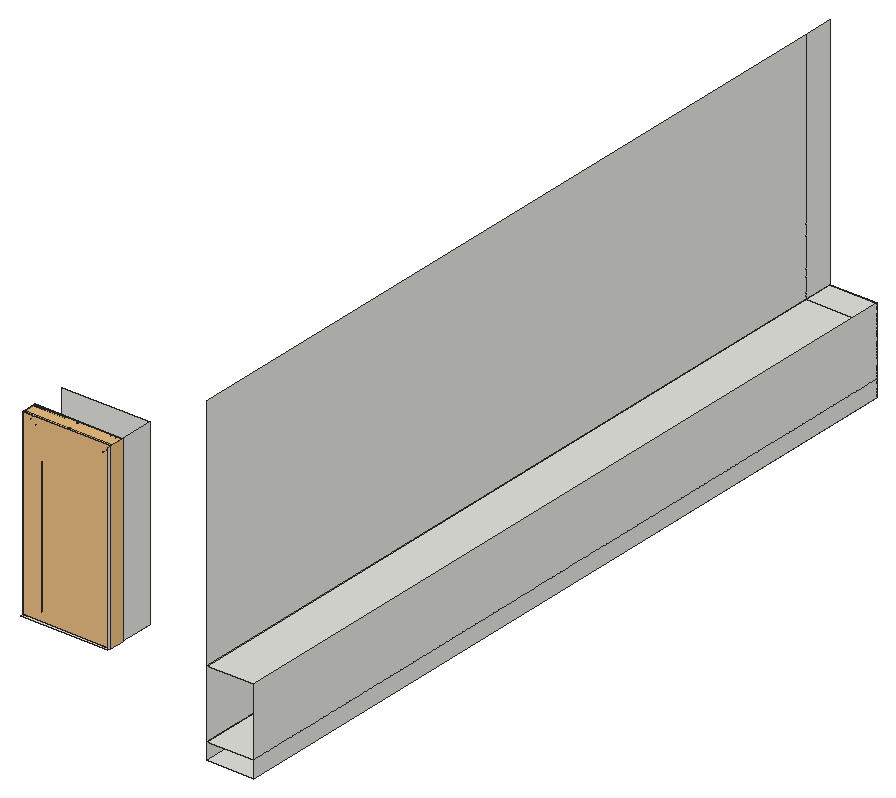
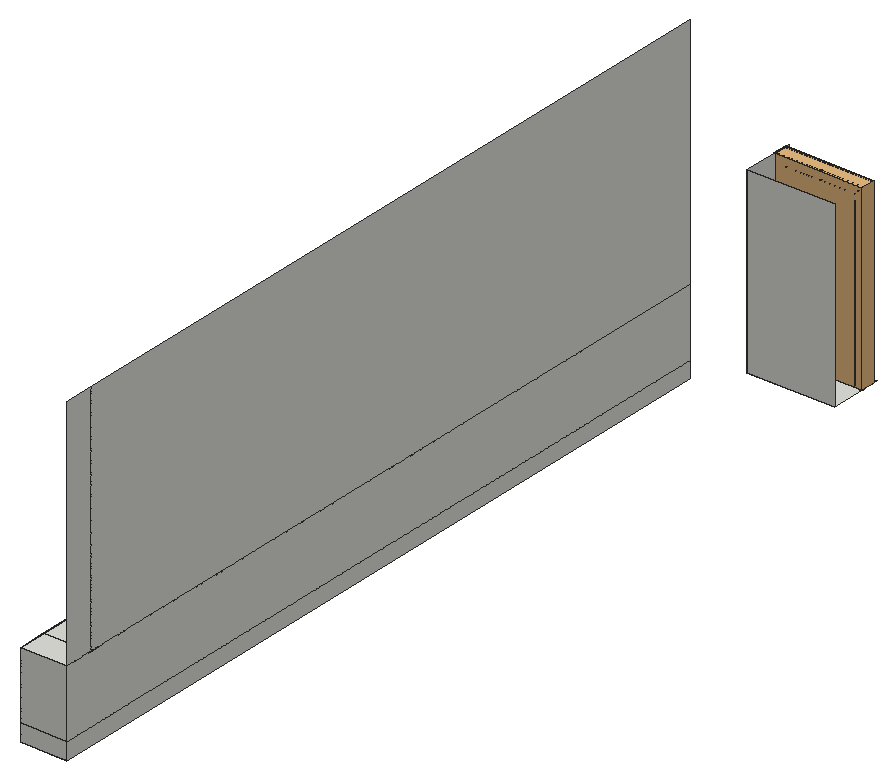
# SketchUp Ruby script. Lengths in inches.
U = 1.inch
M = Sketchup.active_model
def pt(a) = Geom::Point3d.new(a.map { |v| v * U })
def face(e, loops, mat)
  f = e.add_face(loops[0].map { |a| pt(a) })
  loops[1..].each { |l| e.add_face(l.map { |a| pt(a) }).erase! }
  f.material = f.back_material = mat if mat
  f
end
# faces: each face lists its corners as indices into pts; further lists are holes
def faces(e, pts, list, mat = nil) = list.each { |f| face(e, (f[0].is_a?(Array) ? f : [f]).map { |l| l.map { |i| pts[i] } }, mat) }
# xy, xz, yz: faces in a plane at the given z, y or x. An outline is a flat list of corners, or four numbers for a rectangle; further outlines are holes
def ring(l) = l.size == 4 ? [[l[0], l[1]], [l[2], l[1]], [l[2], l[3]], [l[0], l[3]]] : l.each_slice(2).to_a
def flat(e, list, mat, &to3) = list.each { |f| face(e, (f[0].is_a?(Array) ? f : [f]).map { |l| ring(l).map { |u, v| to3.(u, v) } }, mat) }
def xy(e, z, list, mat = nil) = flat(e, list, mat) { |x, y| [x, y, z] }
def xz(e, y, list, mat = nil) = flat(e, list, mat) { |x, z| [x, y, z] }
def yz(e, x, list, mat = nil) = flat(e, list, mat) { |y, z| [x, y, z] }
def lines(e, pts, list) = list.each { |a, b| e.add_line(pt(pts[a]), pt(pts[b])) }
# prism: a flat outline (further loops are holes) pulled along v
def prism(e, loops, v, mat = nil)
  f = face(e, loops, mat); d = Geom::Vector3d.new(v.map { |x| x * U })
  f.pushpull(f.normal.samedirection?(d) ? d.length : -d.length)
end
def box(e, o, s, mat = nil) = prism(e, [[o, [o[0] + s[0], o[1], o[2]], [o[0] + s[0], o[1] + s[1], o[2]], [o[0], o[1] + s[1], o[2]]]], [0, 0, s[2]], mat)
def at(x, y, z, deg = 0) = Geom::Transformation.translation(pt([x, y, z])) * Geom::Transformation.rotation(ORIGIN, Z_AXIS, deg.degrees)
def axes(o, x, y, z) = Geom::Transformation.new([*x, 0, *y, 0, *z, 0, *pt(o).to_a, 1])
def part(name) = M.definitions.add(name)
# library, detail: a bought-in or finely detailed component or shape, given as its bounding box
def library(name, o, s) = part(name).tap { |d| box(d.entities, o, s) }
def detail(e, o, s) = box(e.add_group.entities, o, s)
def put(e, d, t, mat = nil) = e.add_instance(d, t).tap { |i| i.material = mat if mat }
def group(e, t, mat = nil) = e.add_group.tap { |g| g.transformation = t; g.material = mat if mat }.entities
root = M.entities
M.materials.add("Material \#0").color = [86, 53, 35]
M.materials.add("Material \#1").color = [140, 140, 140]
c1 = part("3DGeom~19_Defintion")
xy(c1.entities,0,[[-6.28,-215.79,-994.45,-208.55,-13.52,-208.55],[-994.45,-215.79,-994.45,-208.55,-6.28,-215.79],[-6.28,-215.79,-13.52,-208.55,-13.52,0],[-6.28,-215.79,-13.52,0,-6.28,0],[-13.52,0,-13.52,208.55,-6.28,215.79],
  [-13.52,0,-6.28,215.79,-6.28,0],[-994.45,208.55,-6.28,215.79,-13.52,208.55],[-994.45,208.55,-994.45,215.79,-6.28,215.79]],"Material \#0")
p = [[-13.52,-208.55,0],[-994.45,-208.55,0],[-994.45,-207.81,0.07],[-14.25,-207.81,0.07],[-13.52,-208.55,0],[-14.25,-207.81,0.07],
  [-14.25,0,0.07],[-13.52,0,0],[-13.52,208.55,0],[-14.25,207.81,0.07],[-13.52,208.55,0],[-14.25,207.81,0.07],
  [-994.45,207.81,0.07],[-994.45,208.55,0],[-994.45,-207.21,0.27],[-994.45,-207.21,0.27],[-14.86,-207.21,0.27],[-14.86,-207.21,0.27],
  [-14.86,0,0.27],[-14.86,0,0.27],[-14.86,0,0.27],[-14.86,0,0.27],[-14.86,207.21,0.27],[-14.86,207.21,0.27],
  [-994.45,207.21,0.27],[-994.45,207.21,0.27],[-14.86,-207.21,0.27],[-994.45,-207.21,0.27],[-994.45,-206.74,0.6],[-15.33,-206.74,0.6],
  [-14.86,-207.21,0.27],[-15.33,-206.74,0.6],[-15.33,0,0.6],[-14.86,0,0.27],[-14.86,207.21,0.27],[-15.33,206.74,0.6],
  [-14.86,207.21,0.27],[-15.33,206.74,0.6],[-994.45,206.74,0.6],[-994.45,207.21,0.27],[-994.45,-206.4,1.07],[-15.66,-206.4,1.07],
  [-15.66,-206.4,1.07],[-15.66,0,1.07],[-15.66,206.4,1.07],[-15.66,206.4,1.07],[-994.45,206.4,1.07],[-994.45,-206.2,1.68],
  [-15.86,-206.2,1.68],[-15.86,-206.2,1.68],[-15.86,0,1.68],[-15.86,206.2,1.68],[-15.86,206.2,1.68],[-994.45,206.2,1.68],
  [-994.45,-206.13,2.41],[-15.93,-206.13,2.41],[-15.93,-206.13,2.41],[-15.93,0,2.41],[-15.93,206.13,2.41],[-15.93,206.13,2.41],
  [-994.45,206.13,2.41],[-994.45,-206.13,71.16],[-994.45,-206.22,71.59],[-15.79,-206.28,71.53],[-15.79,-206.28,71.53],[-15.84,0,71.59],
  [-15.93,0,71.16],[-15.79,206.28,71.53],[-15.79,206.28,71.53],[-994.45,206.22,71.59],[-994.45,206.13,71.16],[-15.79,-206.28,71.53],
  [-994.45,-206.48,71.84],[-994.45,-206.9,71.93],[-15.16,-206.9,71.93],[-15.79,-206.28,71.53],[-15.79,-206.28,71.53],[-15.16,-206.9,71.93],
  [-15.16,0,71.93],[-994.45,-206.48,71.84],[-15.59,0,71.84],[-15.79,-206.28,71.53],[-15.59,0,71.84],[-15.79,206.28,71.53],
  [-15.16,206.9,71.93],[-15.59,0,71.84],[-15.79,206.28,71.53],[-994.45,206.48,71.84],[-15.79,206.28,71.53],[-15.16,206.9,71.93],
  [-994.45,206.9,71.93],[-994.45,206.48,71.84],[-15.79,206.28,71.53],[-994.45,-227.27,72.01],[5.41,-227.47,72.33],[4.78,-226.84,71.93],
  [4.78,-226.84,71.93],[5.41,-227.47,72.33],[5.21,0,72.01],[-994.45,-226.84,71.93],[-994.45,-227.27,72.01],[5.21,0,72.01],
  [4.78,0,71.93],[4.78,226.84,71.93],[5.21,0,72.01],[5.21,0,72.01],[5.41,227.47,72.33],[4.78,226.84,71.93],
  [5.41,227.47,72.33],[-994.45,227.27,72.01],[-994.45,227.27,72.01],[-994.45,226.84,71.93],[-994.45,-227.27,72.01],[-994.45,-227.53,72.27],
  [5.41,-227.47,72.33],[5.41,-227.47,72.33],[5.47,0,72.27],[5.21,0,72.01],[5.41,227.47,72.33],[5.41,227.47,72.33],
  [-994.45,227.53,72.27],[-994.45,227.27,72.01],[-994.45,-227.61,72.7],[-994.45,-227.61,74.4375],[-994.45,-227.61,74.4375],[5.55,-227.61,74.4375],
  [5.55,-227.61,74.4375],[5.55,0,74.4375],[5.55,0,72.7],[5.55,227.61,74.4375],[5.55,227.61,74.4375],[-994.45,227.61,74.4375],
  [-994.45,227.61,74.4375],[-994.45,227.61,72.7]]
faces(c1.entities,p,[[0,1,2],[2,3,0],[4,5,6],[6,7,4],[8,7,6],[6,9,8],[10,11,12],[12,13,10],
  [3,2,14],[15,16,3],[5,17,18],[19,6,5],[9,6,20],[21,22,9],[11,23,24],[25,12,11],
  [26,27,28],[28,29,26],[30,31,32],[32,33,30],[34,33,32],[32,35,34],[36,37,38],[38,39,36],
  [29,28,40],[40,41,29],[31,42,43],[43,32,31],[35,32,43],[43,44,35],[37,45,46],[46,38,37],
  [41,40,47],[47,48,41],[42,49,50],[50,43,42],[44,43,50],[50,51,44],[45,52,53],[53,46,45],
  [48,47,54],[54,55,48],[49,56,57],[57,50,49],[51,50,57],[57,58,51],[52,59,60],[60,53,52],
  [61,62,63],[64,65,66],[66,65,67],[68,69,70],[71,72,73],[73,74,75],[76,77,78],[62,79,63],
  [78,80,76],[81,82,65],[83,80,78],[78,84,83],[65,85,86],[68,87,69],[88,89,90],[90,91,92],
  [93,94,95],[96,97,98],[95,99,100],[101,102,96],[103,102,104],[105,106,103],[107,108,109],[110,111,107],
  [112,113,114],[115,116,117],[117,116,118],[119,120,121],[114,122,123],[124,125,114],[113,122,114],[115,126,127],
  [127,128,115],[115,128,116],[118,128,127],[127,129,118],[116,128,118],[119,130,131],[132,133,119],[119,133,120]],"Material \#0")
c2 = part("3DGeom~15_Defintion")
xy(c2.entities,0,[[-961.58,-251.9,-958.5,-248.8125,-961.58,-237.8],[-961.58,-251.9,28.8,-248.8125,-958.5,-248.8125],[-961.58,-251.9,36.25,-251.9,28.8,-248.8125],[36.25,-251.9,19.98,-239.99,28.8,-248.8125],[36.25,-251.9,22.16,-237.8,19.98,-239.99],
  [-958.5,-248.8125,-958.5,-237.8,-961.58,-237.8],[19.98,-239.99,22.16,-237.8,3.36,-223.37],[-958.5,-237.8,-958.5,-223.37,-961.58,-220.28],[-961.58,-237.8,-958.5,-237.8,-961.58,-220.28],[22.16,-237.8,4.64,-220.28,3.36,-223.37],
  [-958.5,-223.37,4.64,-220.28,-961.58,-220.28],[-958.5,-223.37,3.36,-223.37,4.64,-220.28],[5.29,-219.63,8.375,-218.35,5.29,0],[8.375,-218.35,8.375,0,5.29,0],[5.29,0,8.375,0,5.29,219.63],
  [8.375,0,8.375,218.35,5.29,219.63],[8.375,218.35,22.8125,237.15,5.29,219.63],[-961.58,220.28,-958.5,223.37,-961.58,237.8],[-961.58,220.28,3.36,223.37,-958.5,223.37],[-961.58,220.28,4.64,220.28,3.36,223.37],
  [4.64,220.28,19.98,239.99,3.36,223.37],[4.64,220.28,22.16,237.8,19.98,239.99],[-958.5,223.37,-958.5,237.8,-961.58,237.8],[-958.5,237.8,-958.5,248.8125,-961.58,251.9],[-961.58,237.8,-958.5,237.8,-961.58,251.9],
  [22.16,237.8,28.8,248.8125,19.98,239.99],[22.16,237.8,36.25,251.9,28.8,248.8125],[-958.5,248.8125,36.25,251.9,-961.58,251.9],[-958.5,248.8125,28.8,248.8125,36.25,251.9]],"Material \#0")
xy(c2.entities,7.48,[[-962.79,-238.36,23.37,-238.36,-962.79,-219.67],[23.37,-238.36,4.67,-219.67,-962.79,-219.67],[23.37,-238.36,23.37,0,4.67,-219.67],[4.67,-219.67,23.37,0,4.67,0],[23.37,0,23.37,238.36,4.67,219.67],
  [4.67,0,23.37,0,4.67,219.67],[-962.79,219.67,23.37,238.36,-962.79,238.36],[-962.79,219.67,4.67,219.67,23.37,238.36]],"Material \#0")
xy(c2.entities,63.5625,[[-962.79,-238.36,-962.79,-219.67,4.67,-219.67],[-962.79,-238.36,4.67,-219.67,23.37,-238.36],[23.37,-238.36,4.67,-219.67,23.37,0],[4.67,-219.67,4.67,0,23.37,0],[23.37,0,4.67,219.67,23.37,238.36],
  [4.67,0,4.67,219.67,23.37,0],[-962.79,219.67,-962.79,238.36,4.67,219.67],[4.67,219.67,-962.79,238.36,23.37,238.36]],"Material \#0")
xy(c2.entities,69.64,[[-962.79,-219.62,4.63,-219.62,-962.79,-200.32],[4.63,-219.62,-14.68,-200.32,-962.79,-200.32],[4.63,-219.62,4.63,0,-14.68,-200.32],[-14.68,-200.32,4.63,0,-14.68,0],[-14.68,0,4.63,0,-14.68,200.32],
  [4.63,0,4.63,219.62,-14.68,200.32],[-962.79,200.32,-14.68,200.32,4.63,219.62],[-962.79,200.32,4.63,219.62,-962.79,219.62]],"Material \#0")
xy(c2.entities,71.04,[[-961.58,-251.9,-958.5,-248.8125,28.8,-248.8125],[-961.58,-251.9,-961.58,-237.8,-958.5,-248.8125],[-961.58,-251.9,28.8,-248.8125,36.25,-251.9],[36.25,-251.9,19.98,-239.99,22.16,-237.8],[36.25,-251.9,28.8,-248.8125,19.98,-239.99],
  [-958.5,-248.8125,-961.58,-237.8,-958.5,-237.8],[19.98,-239.99,3.36,-223.37,22.16,-237.8],[-958.5,-237.8,-961.58,-220.28,-958.5,-223.37],[-961.58,-237.8,-961.58,-220.28,-958.5,-237.8],[22.16,-237.8,3.36,-223.37,4.64,-220.28],
  [-958.5,-223.37,-961.58,-220.28,4.64,-220.28],[-958.5,-223.37,4.64,-220.28,3.36,-223.37],[5.29,-219.63,5.29,0,8.375,-218.35],[8.375,-218.35,5.29,0,8.375,0],[5.29,0,5.29,219.63,8.375,0],
  [8.375,0,5.29,219.63,8.375,218.35],[8.375,218.35,5.29,219.63,22.8125,237.15],[-961.58,220.28,-958.5,223.37,3.36,223.37],[-961.58,220.28,-961.58,237.8,-958.5,223.37],[-961.58,220.28,3.36,223.37,4.64,220.28],
  [4.64,220.28,3.36,223.37,19.98,239.99],[4.64,220.28,19.98,239.99,22.16,237.8],[-958.5,223.37,-961.58,237.8,-958.5,237.8],[-958.5,237.8,-961.58,251.9,-958.5,248.8125],[-961.58,237.8,-961.58,251.9,-958.5,237.8],
  [22.16,237.8,19.98,239.99,28.8,248.8125],[22.16,237.8,28.8,248.8125,36.25,251.9],[-958.5,248.8125,-961.58,251.9,36.25,251.9],[-958.5,248.8125,36.25,251.9,28.8,248.8125]],"Material \#0")
xz(c2.entities,-238.36,[[-962.79,63.5625,23.37,63.5625,23.37,72.07],[-962.79,63.5625,23.37,72.07,-962.79,72.07]],"Material \#0")
xz(c2.entities,-219.67,[[-962.79,7.48,4.67,7.48,-962.79,63.5625],[4.67,7.48,4.67,63.5625,-962.79,63.5625]],"Material \#0")
xz(c2.entities,219.67,[[-962.79,7.48,-962.79,63.5625,4.67,7.48],[4.67,7.48,-962.79,63.5625,4.67,63.5625]],"Material \#0")
xz(c2.entities,238.36,[[-962.79,63.5625,-962.79,72.07,23.37,72.07],[-962.79,63.5625,23.37,72.07,23.37,63.5625]],"Material \#0")
yz(c2.entities,4.67,[[-219.67,7.48,0,7.48,-219.67,63.5625],[0,7.48,0,63.5625,-219.67,63.5625],[0,7.48,219.67,63.5625,0,63.5625],[0,7.48,219.67,7.48,219.67,63.5625]],"Material \#0")
yz(c2.entities,23.37,[[-238.36,63.5625,0,63.5625,-238.36,72.07],[0,63.5625,0,72.07,-238.36,72.07],[0,63.5625,238.36,63.5625,238.36,72.07],[0,63.5625,238.36,72.07,0,72.07]],"Material \#0")
p = [[36.9,-251.24,0],[37.21,0,-0.16],[34.125,0,-0.14],[36.9,251.24,0],[33.83,243.81,0.02],[33.83,-243.8,0.02],
  [22.8125,-237.15,0],[24.99,-234.97,-0.01],[5.375,-220.37,0],[23.37,-238.36,7.48],[4.67,-219.67,7.48],[4.67,-219.67,7.48],
  [23.37,-238.36,7.48],[23.37,-238.36,0],[4.67,-219.67,7.48],[23.37,-238.36,0],[5.375,-220.37,0],[5.375,-220.37,0],
  [23.37,-238.36,0],[5.29,-219.63,0],[8.375,-218.35,0],[-15.36,-199.64,1.62],[4.67,-219.67,7.48],[5.375,-220.37,0],
  [-13.8,-201.19,0.06],[5.375,-220.37,0],[5.375,-220.37,0],[-14.84,-200.15,0.58],[5.375,-220.37,0],[-13.8,-201.19,0.06],
  [-6.08,-208.92,0],[5.375,-220.37,0],[-13.8,-201.19,0.06],[-6.08,-208.92,0],[-13.8,-201.19,0.06],[5.375,-220.37,0],
  [-6.08,-208.92,0],[-13.8,-201.19,0.06],[-13.09,-201.91,0],[-6.08,-208.92,0],[-13.09,-201.91,0],[-13.8,-201.19,0.06],
  [-15.36,199.64,1.62],[4.67,219.67,7.48],[5.375,220.37,0],[-13.8,201.19,0.06],[5.375,220.37,0],[5.375,220.37,0],
  [4.67,219.67,7.48],[-14.84,200.15,0.58],[5.375,220.37,0],[-13.8,201.19,0.06],[-6.08,208.92,0],[-13.09,201.91,0],
  [-13.8,201.19,0.06],[-6.08,208.92,0],[-13.8,201.19,0.06],[5.375,220.37,0],[-6.08,208.92,0],[5.375,220.37,0],
  [-13.8,201.19,0.06],[-6.08,208.92,0],[-13.8,201.19,0.06],[-13.09,201.91,0],[8.375,218.35,0],[24.99,234.97,-0.01],
  [22.8125,237.15,0],[23.37,238.36,7.48],[23.37,238.36,0],[23.37,238.36,0],[5.375,220.37,0],[5.375,220.37,0],
  [23.37,238.36,7.48],[4.67,219.67,7.48],[5.375,220.37,0],[23.37,238.36,0],[23.37,238.36,7.48],[-13.8,-201.19,0.06],
  [-14.84,-200.15,0.58],[-14.38,-200.61,0.26],[-13.8,-201.19,0.06],[-13.8,-201.19,0.06],[-14.38,-200.61,0.26],[-13.8,201.19,0.06],
  [-14.84,200.15,0.58],[-13.8,201.19,0.06],[-14.38,200.61,0.26],[-14.38,200.61,0.26],[-13.8,201.19,0.06],[4.63,-219.62,69.64],
  [4.63,-219.62,69.64],[-15.42,-199.57,9.43],[-15.36,-199.64,1.62],[-15.16,-199.83,1.04],[-15.16,-199.83,1.04],[-15.16,199.83,1.04],
  [-15.36,199.64,1.62],[-15.16,199.83,1.04],[-15.42,199.57,9.43],[4.63,219.62,69.64],[4.67,219.67,7.48],[4.63,219.62,69.64],
  [4.63,-219.62,69.64],[4.67,-219.67,63.5625],[4.67,-219.67,63.5625],[4.67,-219.67,7.48],[-15.28,-199.71,69.25],[4.63,-219.62,69.64],
  [-15.42,-199.57,9.43],[-15.28,-199.71,69.25],[-15.42,-199.57,2.34],[-15.42,-199.57,2.34],[-15.42,199.57,2.34],[-15.42,199.57,9.43],
  [-15.28,199.71,69.25],[-15.28,199.71,69.25],[4.63,219.62,69.64],[4.63,219.62,69.64],[4.67,219.67,63.5625],[4.67,219.67,63.5625],
  [-15.42,199.57,2.34],[4.67,-219.67,63.5625],[4.63,-219.62,69.64],[4.67,219.67,7.48],[4.67,219.67,63.5625],[4.63,219.62,69.64],
  [4.63,-219.62,69.64],[-15.28,-199.71,69.25],[-15.28,-199.71,69.25],[-15.42,-199.57,48.99],[-15.42,-199.57,48.99],[-15.28,-199.71,69.25],
  [-15.42,199.57,48.99],[-15.28,199.71,69.25],[-15.28,199.71,69.25],[-15.42,199.57,48.99],[4.63,219.62,69.64],[4.63,-219.62,69.64],
  [23.37,-238.36,72.07],[4.67,-219.67,63.5625],[4.67,-219.67,63.5625],[23.37,-238.36,63.5625],[23.37,-238.36,72.07],[4.67,-219.67,63.5625],
  [5.24,-220.23,70.03],[23.37,-238.36,72.07],[23.37,-238.36,63.5625],[4.67,-219.67,63.5625],[4.67,-219.67,63.5625],[4.63,-219.62,69.64],
  [4.63,219.62,69.64],[23.37,238.36,72.07],[4.67,219.67,63.5625],[4.67,219.67,63.5625],[5.24,220.23,70.03],[4.63,219.62,69.64],
  [23.37,238.36,63.5625],[4.67,219.67,63.5625],[4.67,219.67,63.5625],[23.37,238.36,63.5625],[23.37,238.36,72.07],[4.67,219.67,63.5625],
  [23.37,238.36,72.07],[4.63,-219.62,69.64],[-14.68,-200.32,69.64],[-15.28,-199.71,69.25],[-15.28,-199.71,69.25],[-14.68,-200.32,69.64],
  [4.63,-219.62,69.64],[-15.28,199.71,69.25],[-14.68,200.32,69.64],[4.63,219.62,69.64],[4.63,219.62,69.64],[-14.68,200.32,69.64],
  [4.63,-219.62,69.64],[5.24,-220.23,70.03],[23.37,-238.36,72.07],[4.63,219.62,69.64],[5.24,220.23,70.03],[5.375,-220.37,72.07],
  [5.375,-220.37,72.07],[23.37,-238.36,72.07],[5.375,220.37,72.07],[23.37,238.36,72.07],[5.375,220.37,72.07],[33.83,-243.8,71.03],
  [36.9,-251.24,71.04],[22.8125,-237.15,71.04],[34.125,0,71.19],[37.21,0,71.2],[24.99,-234.97,71.05],[5.29,-219.63,71.04],
  [8.375,-218.35,71.04],[33.83,243.81,71.03],[36.9,251.24,71.04],[22.8125,237.15,71.04],[24.99,234.97,71.05],[8.375,218.35,71.04]]
faces(c2.entities,p,[[0,1,2],[1,3,4],[4,2,1],[2,5,0],[6,0,5],[5,7,6],[8,9,10],[11,12,13],
  [14,15,16],[17,18,9],[19,6,7],[7,20,19],[21,22,23],[24,21,25],[26,10,27],[28,27,29],
  [30,31,32],[33,34,35],[36,37,38],[39,40,41],[42,43,44],[45,42,46],[47,48,49],[50,49,51],
  [52,53,54],[55,56,57],[58,59,60],[61,62,63],[64,65,66],[43,67,68],[43,69,70],[71,72,73],
  [74,75,76],[3,66,65],[65,4,3],[77,78,21],[27,79,80],[81,82,78],[83,84,42],[85,86,84],
  [49,87,88],[10,89,27],[90,91,27],[92,93,27],[91,92,27],[78,94,21],[84,95,42],[96,97,49],
  [98,96,49],[99,98,49],[100,101,49],[21,102,103],[21,104,105],[21,106,107],[21,108,109],[91,110,92],
  [21,111,108],[42,112,113],[42,113,114],[42,115,116],[42,117,118],[42,119,43],[98,120,96],[10,121,122],
  [123,124,125],[126,127,91],[128,129,91],[108,130,131],[113,132,133],[134,135,98],[136,134,98],[137,138,139],
  [140,141,142],[143,142,144],[145,146,147],[148,144,149],[150,151,152],[153,154,155],[151,156,157],[158,159,160],
  [161,162,154],[163,164,165],[166,167,168],[169,170,171],[172,173,134],[174,175,176],[177,178,151],[142,179,144],
  [175,180,181],[178,182,151],[183,184,154],[185,186,187],[186,185,188],[188,189,186],[187,190,185],[190,187,191],
  [191,192,190],[189,188,193],[193,194,189],[195,196,197],[196,195,194],[194,193,196]],"Material \#0")
c3 = part("3DGeom~22_Defintion")
xz(c3.entities,-210.625,[[-1016.13,2.47,-1016.13,9.96,-16.28,2.47],[-16.28,2.47,-1016.13,9.96,-16.28,9.96],[-1016.13,9.96,-1016.13,51.7,-16.28,51.7],[-1016.13,9.96,-16.28,51.7,-16.28,9.96],[-1016.13,51.7,-1016.13,72.71,-16.28,51.7]],"Material \#0")
xz(c3.entities,210.625,[[-1016.13,2.47,-16.28,2.47,-1016.13,9.96],[-16.28,2.47,-16.28,9.96,-1016.13,9.96],[-1016.13,9.96,-16.28,51.7,-1016.13,51.7],[-1016.13,9.96,-16.28,9.96,-16.28,51.7],[-1016.13,51.7,-16.28,51.7,-1016.13,72.71]],"Material \#0")
yz(c3.entities,-16.28,[[-210.625,2.47,-210.625,9.96,0,9.96],[-210.625,2.47,0,9.96,0,2.47],[0,2.47,0,9.96,210.625,2.47],[210.625,2.47,0,9.96,210.625,9.96],[-210.625,9.96,-210.625,51.7,0,51.7],
  [-210.625,9.96,0,51.7,0,9.96],[0,9.96,0,51.7,210.625,9.96],[210.625,9.96,0,51.7,210.625,51.7],[-210.625,51.7,0,72.71,0,51.7],[0,51.7,0,72.71,210.625,51.7]],"Material \#0")
p = [[-1016.13,-210.625,72.71],[-16.13,-210.77,73.09],[-16.28,-210.625,51.7],[-16.28,-210.625,51.7],[-16.13,-210.77,73.09],[-16.28,0,72.71],
  [-16.13,210.77,73.09],[-16.28,210.625,51.7],[-16.28,210.625,51.7],[-16.13,210.77,73.09],[-1016.13,210.625,72.71]]
faces(c3.entities,p,[[0,1,2],[3,4,5],[5,6,7],[8,9,10]],"Material \#0")
c4 = library("3DGeom~16_Defintion",[-962.62,-252.34,-11.22],[1000,504.68,93.46])
c5 = part("3DGeom~17_Defintion")
yz(c5.entities,-1908.8,[[-436.03,-21.87,-436.73,-21.5,-435.91,-21.83],[436.03,-21.87,435.91,-21.83,436.73,-21.5],[-435.91,-21.83,-436.73,-21.5,-436.15,-21.125],[-435.91,-21.83,-436.15,-21.125,-435.87,-21.72],[435.91,-21.83,435.87,-21.72,436.15,-21.125],
  [435.91,-21.83,436.15,-21.125,436.73,-21.5],[-436.73,-21.5,-484.73,-21.37,-436.15,-1.11],[-471.46,-21.5,-484.73,-21.37,-436.73,-21.5],[-477.2,-21.5,-484.73,-21.37,-471.46,-21.5],[-481.82,-21.5,-484.73,-21.37,-477.2,-21.5],
  [-436.73,-21.5,-436.15,-1.11,-436.15,-21.125],[436.73,-21.5,436.15,-21.125,471.46,-21.5],[471.46,-21.5,436.15,-21.125,477.2,-21.5],[477.2,-21.5,436.15,-21.125,499.98,-0.85],[477.2,-21.5,499.98,-0.85,481.82,-21.5],
  [481.82,-21.5,487.35,-21,484.73,-21.37],[481.82,-21.5,491.8,-19.52,487.35,-21],[481.82,-21.5,497.64,-13.67,491.8,-19.52],[481.82,-21.5,499.98,-0.85,497.64,-13.67],[-484.73,-21.37,-498.5,-11.58,-499.84,-0.37],
  [-484.73,-21.37,-499.84,-0.37,-499.4,-0.5],[-484.73,-21.37,-499.4,-0.5,-436.15,-1.11],[-484.73,-21.37,-493.63,-18.42,-498.5,-11.58],[-484.73,-21.37,-489.71,-20.375,-493.63,-18.42],[-484.73,-21.37,-487.35,-21,-489.71,-20.375],
  [436.15,-21.125,436.15,-1.11,436.73,-0.74],[436.15,-21.125,436.73,-0.74,499.98,-0.85],[487.35,-21,491.8,-19.52,489.71,-20.375],[-489.71,-20.375,-491.8,-19.52,-493.63,-18.42],[491.8,-19.52,495.21,-17.08,493.63,-18.42],
  [491.8,-19.52,497.64,-13.67,495.21,-17.08],[-493.63,-18.42,-496.54,-15.5,-498.5,-11.58],[-493.63,-18.42,-495.21,-17.08,-496.54,-15.5],[495.21,-17.08,497.64,-13.67,496.54,-15.5],[-496.54,-15.5,-497.64,-13.67,-498.5,-11.58],
  [497.64,-13.67,499.125,-9.22,498.5,-11.58],[497.64,-13.67,499.625,-3.69,499.125,-9.22],[497.64,-13.67,499.98,-0.85,499.625,-3.69],[-498.5,-11.58,-499.625,-3.69,-499.84,-0.37],[-498.5,-11.58,-499.5,-6.6,-499.625,-3.69],
  [-498.5,-11.58,-499.125,-9.22,-499.5,-6.6],[499.125,-9.22,499.625,-3.69,499.5,-6.6],[-499.625,-3.69,-499.98,-0.85,-500,-0.52],[-499.625,-3.69,-500,-0.52,-499.84,-0.37],[-436.15,-1.11,-499.4,-0.5,-471.46,-0.74],
  [-436.15,-1.11,-471.46,-0.74,-436.73,-0.74],[-436.15,-1.11,-436.73,-0.74,-435.91,-0.41],[-436.15,-1.11,-435.91,-0.41,-435.87,-0.52],[436.15,-1.11,435.87,-0.52,435.91,-0.41],[436.15,-1.11,435.91,-0.41,436.73,-0.74],
  [499.98,-0.85,436.73,-0.74,471.46,-0.74],[499.98,-0.85,471.46,-0.74,499.4,-0.5],[499.98,-0.85,499.4,-0.5,499.96,-0.41],[499.98,-0.85,499.96,-0.41,500,-0.52],[-436.73,-0.74,-436.03,-0.37,-435.91,-0.41],
  [436.73,-0.74,435.91,-0.41,436.03,-0.37],[-500,-0.52,-499.96,-0.41,-499.84,-0.37],[499.4,-0.5,499.84,-0.37,499.96,-0.41],[-499.84,141.21,-499.96,141.25,-499.4,141.35],[-436.03,141.21,-436.73,141.59,-435.91,141.25],
  [436.03,141.21,435.91,141.25,436.73,141.59],[499.84,141.21,484.73,162.21,498.5,152.42],[499.84,141.21,499.4,141.35,484.73,162.21],[499.84,141.21,498.5,152.42,499.625,144.53],[499.84,141.21,499.625,144.53,500,141.37],
  [499.84,141.21,500,141.37,499.96,141.25],[-499.96,141.25,-500,141.37,-499.98,141.69],[-499.96,141.25,-499.98,141.69,-499.4,141.35],[-435.91,141.25,-436.73,141.59,-436.15,141.96],[-435.91,141.25,-436.15,141.96,-435.87,141.37],
  [435.91,141.25,435.87,141.37,436.15,141.96],[435.91,141.25,436.15,141.96,436.73,141.59],[-499.4,141.35,-499.98,141.69,-471.46,141.59],[499.4,141.35,436.15,141.96,484.73,162.21],[499.4,141.35,471.46,141.59,436.15,141.96],
  [500,141.37,499.625,144.53,499.98,141.69],[-436.73,141.59,-499.98,141.69,-436.15,161.97],[-471.46,141.59,-499.98,141.69,-436.73,141.59],[-436.73,141.59,-436.15,161.97,-436.15,141.96],[436.73,141.59,436.15,141.96,471.46,141.59],
  [-499.98,141.69,-477.2,162.34,-436.15,161.97],[-499.98,141.69,-481.82,162.34,-477.2,162.34],[-499.98,141.69,-497.64,154.51,-481.82,162.34],[-499.98,141.69,-499.625,144.53,-497.64,154.51],[436.15,141.96,436.15,161.97,436.73,162.34],
  [436.15,141.96,436.73,162.34,484.73,162.21],[-499.625,144.53,-499.125,150.07,-497.64,154.51],[-499.625,144.53,-499.5,147.44,-499.125,150.07],[499.625,144.53,498.5,152.42,499.5,147.44],[499.5,147.44,498.5,152.42,499.125,150.07],
  [-499.125,150.07,-498.5,152.42,-497.64,154.51],[498.5,152.42,484.73,162.21,493.63,159.26],[498.5,152.42,493.63,159.26,496.54,156.34],[498.5,152.42,496.54,156.34,497.64,154.51],[-497.64,154.51,-491.8,160.36,-481.82,162.34],
  [-497.64,154.51,-495.21,157.92,-491.8,160.36],[-497.64,154.51,-496.54,156.34,-495.21,157.92],[496.54,156.34,493.63,159.26,495.21,157.92],[-495.21,157.92,-493.63,159.26,-491.8,160.36],[493.63,159.26,484.73,162.21,489.71,161.22],
  [493.63,159.26,489.71,161.22,491.8,160.36],[-491.8,160.36,-487.35,161.84,-481.82,162.34],[-491.8,160.36,-489.71,161.22,-487.35,161.84],[489.71,161.22,484.73,162.21,487.35,161.84],[-487.35,161.84,-484.73,162.21,-481.82,162.34],
  [-436.15,161.97,-477.2,162.34,-471.46,162.34],[-436.15,161.97,-471.46,162.34,-436.73,162.34],[-436.15,161.97,-436.73,162.34,-435.91,162.68],[-436.15,161.97,-435.91,162.68,-435.87,162.56],[436.15,161.97,435.87,162.56,435.91,162.68],
  [436.15,161.97,435.91,162.68,436.73,162.34],[484.73,162.21,436.73,162.34,471.46,162.34],[484.73,162.21,471.46,162.34,477.2,162.34],[484.73,162.21,477.2,162.34,481.82,162.34],[-436.73,162.34,-436.03,162.72,-435.91,162.68],
  [436.73,162.34,435.91,162.68,436.03,162.72]],"Material \#0")
c6 = part("3DGeom~18_Defintion")
xz(c6.entities,-241.71,[[-976.3,0,23.7,0,23.7,7.58],[-976.3,0,23.7,7.58,-976.3,7.58]],"Material \#0")
xz(c6.entities,241.71,[[-976.3,0,-976.3,7.58,23.7,7.58],[-976.3,0,23.7,7.58,23.7,0]],"Material \#0")
yz(c6.entities,23.7,[[-241.71,0,0,0,-241.71,7.58],[0,0,0,7.58,-241.71,7.58],[0,0,241.71,0,241.71,7.58],[0,0,241.71,7.58,0,7.58]],"Material \#0")
c7 = part("3DGeom~20_Defintion")
xy(c7.entities,0,[[-976.3,-241.71,-976.3,-223.46,23.7,-241.71],[23.7,-241.71,-976.3,-223.46,5.45,-223.46],[23.7,-241.71,5.45,-223.46,5.45,0],[23.7,-241.71,5.45,0,23.7,0],[-976.3,-223.46,-976.3,-211.85,5.45,-223.46],
  [5.45,-223.46,-976.3,-211.85,-6.16,-211.85],[5.45,-223.46,-6.16,-211.85,-6.16,0],[5.45,-223.46,-6.16,0,5.45,0],[-6.16,0,-6.16,211.85,5.45,223.46],[-6.16,0,5.45,223.46,5.45,0],
  [5.45,0,23.7,241.71,23.7,0],[5.45,0,5.45,223.46,23.7,241.71],[-976.3,211.85,-976.3,223.46,5.45,223.46],[-976.3,211.85,5.45,223.46,-6.16,211.85],[-976.3,223.46,-976.3,241.71,23.7,241.71],
  [-976.3,223.46,23.7,241.71,5.45,223.46]],"Material \#0")
xy(root,-42.8125,[[424.88,114.8125,448.63,508.6875]])
xy(root,-34.3125,[[424.88,114.8125,448.63,508.6875]])
xy(root,-10.53,[[330.35,114.8125,374.48,141.3125]])
xy(root,0,[[424.88,114.8125,448.63,493.6875],[424.88,493.6875,448.63,508.6875]])
xz(root,118.74,[[337.22,27.35,337.35,27.37,337.35,27.38],[337.22,27.35,337.35,27.38,337.22,27.37],[337.35,27.37,337.47,27.4,337.47,27.41],[337.35,27.37,337.47,27.41,337.35,27.38],[337.47,27.4,337.58,27.46,337.58,27.47],
  [337.47,27.4,337.58,27.47,337.47,27.41],[337.58,27.46,337.68,27.53,337.68,27.54],[337.58,27.46,337.68,27.54,337.58,27.47],[337.68,27.53,337.76,27.63,337.68,27.54],[337.68,27.53,337.77,27.62,337.76,27.63],
  [337.22,27.56,337.26,27.56,337.26,27.57],[337.22,27.56,337.26,27.57,337.22,27.57],[337.26,27.56,337.3,27.57,337.3,27.58],[337.26,27.56,337.3,27.58,337.26,27.57],[337.3,27.57,337.33,27.6,337.3,27.58],
  [337.3,27.57,337.34,27.59,337.33,27.6],[337.34,27.59,337.37,27.625,337.33,27.6],[337.34,27.59,337.375,27.61,337.37,27.625],[337.375,27.61,337.39,27.65,337.37,27.625],[337.375,27.61,337.4,27.64,337.39,27.65],
  [337.4,27.64,337.41,27.69,337.39,27.65],[337.4,27.64,337.43,27.68,337.41,27.69],[337.43,27.68,337.43,27.72,337.41,27.69],[337.44,27.72,337.45,27.76,337.44,27.76],[337.44,27.76,337.45,27.76,337.45,27.8],
  [337.45,27.76,337.46,27.8,337.45,27.8],[337.45,27.8,337.46,27.8,337.44,27.85],[337.44,27.85,337.45,27.85,337.43,27.89],[337.43,27.89,337.44,27.89,337.41,27.92],[337.44,27.89,337.43,27.93,337.41,27.92],
  [337.41,27.92,337.43,27.93,337.39,27.96],[337.43,27.93,337.4,27.97,337.39,27.96],[337.39,27.96,337.4,27.97,337.37,27.99],[337.4,27.97,337.375,28,337.37,27.99],[337.37,27.99,337.375,28,337.33,28.01],
  [337.375,28,337.34,28.02,337.33,28.01],[337.33,28.01,337.34,28.02,337.3,28.03],[337.34,28.02,337.3,28.04,337.3,28.03],[337.3,28.03,337.3,28.04,337.26,28.04],[337.22,28.04,337.26,28.04,337.26,28.05],
  [337.22,28.04,337.26,28.05,337.22,28.05],[337.26,28.04,337.3,28.04,337.26,28.05]],"Material \#1")
xz(root,141.3125,[[330.35,-10.53,374.48,81.34]])
xz(root,508.6875,[[424.88,-42.8125,448.63,-34.3125],[424.88,-34.3125,448.63,0]])
yz(root,374.48,[[114.8125,-10.53,141.3125,81.34]])
yz(root,424.88,[[114.8125,-42.8125,508.6875,-34.3125],[114.8125,-34.3125,508.6875,0],[114.8125,0,493.6875,120],[493.6875,0,508.6875,120]])
yz(root,448.63,[[114.8125,-42.8125,508.6875,-34.3125],[114.8125,-34.3125,508.6875,0]])
put(root,c1,axes([352.49,123.125,77.91],[0,0,0.08893],[0.08547,0,0],[0,-0.0777,0]),"Material \#0")
put(root,c2,axes([352.49,123.125,77.91],[0,0,0.09186],[0.08828,0,0],[0,-0.08026,0]),"Material \#0")
put(root,c3,axes([352.49,123.125,77.91],[0,0,0.08704],[0.08365,0,0],[0,-0.07604,0]),"Material \#0")
put(root,c4,axes([352.49,123.125,77.91],[0,0,0.09187],[0.0883,0,0],[0,-0.08027,0]),"Material \#0")
put(root,c5,axes([352.49,123.125,77.91],[0,0,0.04633],[0.04453,0,0],[0,-0.04048,0]),"Material \#0")
put(root,c6,axes([352.49,123.125,77.91],[0,0,0.09059],[0.08706,0,0],[0,-0.07915,0]),"Material \#0")
put(root,c7,axes([352.49,123.125,77.91],[0,0,0.09059],[0.08706,0,0],[0,-0.07915,0]),"Material \#0")
